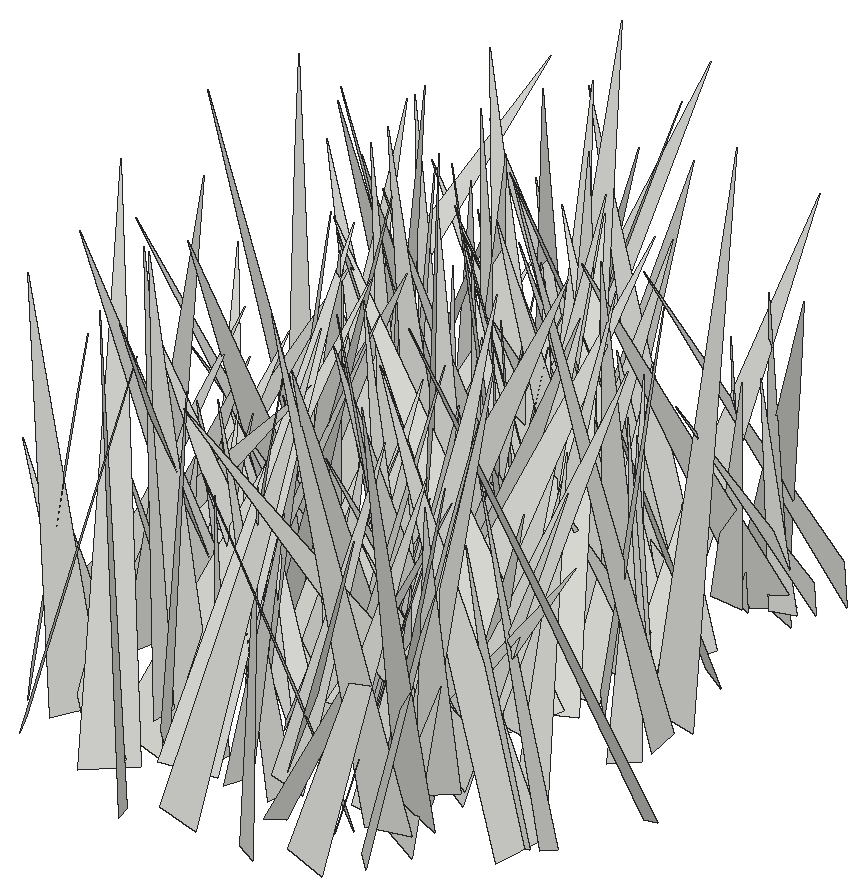
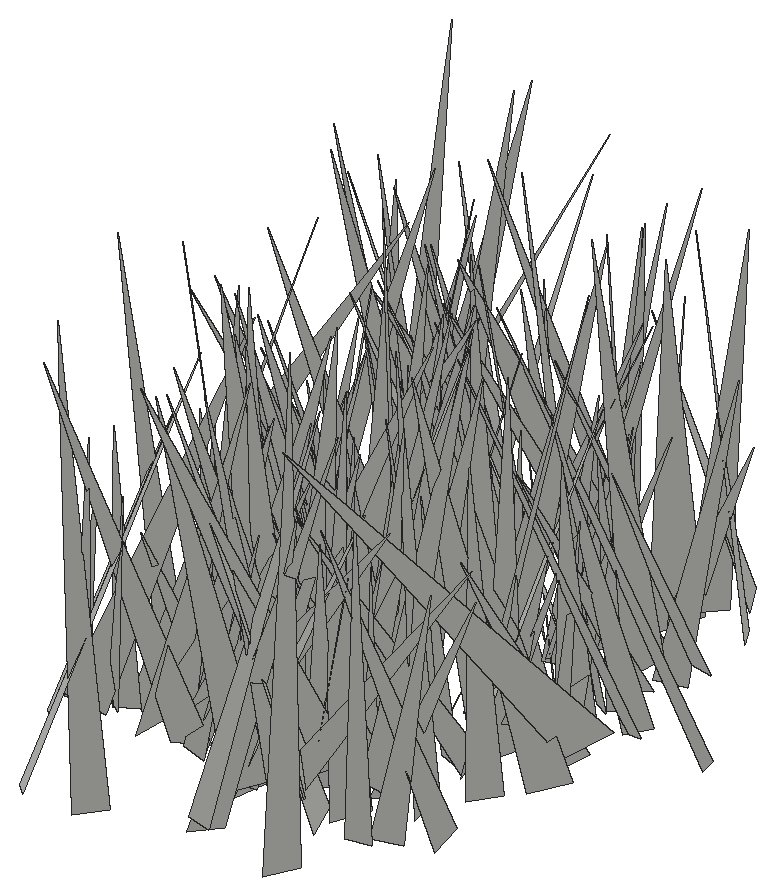
# SketchUp Ruby script. Lengths in inches.
U = 1.inch
M = Sketchup.active_model
def pt(a) = Geom::Point3d.new(a.map { |v| v * U })
def face(e, loops, mat)
  f = e.add_face(loops[0].map { |a| pt(a) })
  loops[1..].each { |l| e.add_face(l.map { |a| pt(a) }).erase! }
  f.material = f.back_material = mat if mat
  f
end
# faces: each face lists its corners as indices into pts; further lists are holes
def faces(e, pts, list, mat = nil) = list.each { |f| face(e, (f[0].is_a?(Array) ? f : [f]).map { |l| l.map { |i| pts[i] } }, mat) }
# xy, xz, yz: faces in a plane at the given z, y or x. An outline is a flat list of corners, or four numbers for a rectangle; further outlines are holes
def ring(l) = l.size == 4 ? [[l[0], l[1]], [l[2], l[1]], [l[2], l[3]], [l[0], l[3]]] : l.each_slice(2).to_a
def flat(e, list, mat, &to3) = list.each { |f| face(e, (f[0].is_a?(Array) ? f : [f]).map { |l| ring(l).map { |u, v| to3.(u, v) } }, mat) }
def xy(e, z, list, mat = nil) = flat(e, list, mat) { |x, y| [x, y, z] }
def xz(e, y, list, mat = nil) = flat(e, list, mat) { |x, z| [x, y, z] }
def yz(e, x, list, mat = nil) = flat(e, list, mat) { |y, z| [x, y, z] }
def lines(e, pts, list) = list.each { |a, b| e.add_line(pt(pts[a]), pt(pts[b])) }
# prism: a flat outline (further loops are holes) pulled along v
def prism(e, loops, v, mat = nil)
  f = face(e, loops, mat); d = Geom::Vector3d.new(v.map { |x| x * U })
  f.pushpull(f.normal.samedirection?(d) ? d.length : -d.length)
end
def box(e, o, s, mat = nil) = prism(e, [[o, [o[0] + s[0], o[1], o[2]], [o[0] + s[0], o[1] + s[1], o[2]], [o[0], o[1] + s[1], o[2]]]], [0, 0, s[2]], mat)
def at(x, y, z, deg = 0) = Geom::Transformation.translation(pt([x, y, z])) * Geom::Transformation.rotation(ORIGIN, Z_AXIS, deg.degrees)
def axes(o, x, y, z) = Geom::Transformation.new([*x, 0, *y, 0, *z, 0, *pt(o).to_a, 1])
def part(name) = M.definitions.add(name)
# library, detail: a bought-in or finely detailed component or shape, given as its bounding box
def library(name, o, s) = part(name).tap { |d| box(d.entities, o, s) }
def detail(e, o, s) = box(e.add_group.entities, o, s)
def put(e, d, t, mat = nil) = e.add_instance(d, t).tap { |i| i.material = mat if mat }
def group(e, t, mat = nil) = e.add_group.tap { |g| g.transformation = t; g.material = mat if mat }.entities
root = M.entities
c1 = part("fur_instance\#9")
p = [[0.8125,0,1.79],[0.67,-0.02,1.48],[0,-0.11,0],[0,0.11,0]]
faces(c1.entities,p,[[0,1,2,3]])
put(root,c1,axes([100.4,143.04,-28.22],[-2.55012,3.64542,1.48438],[3.93085,2.44958,0.73729],[0.20222,-1.64502,4.38733]))
put(root,c1,axes([97.49,134.62,-27.1],[1.64693,-4.65446,0.85777],[-4.4282,-1.19483,2.01879],[1.67056,1.42146,4.50564]))
put(root,c1,axes([99.8,130.2,-28.22],[2.45481,-4.16097,0.8917],[-4.06011,-2.59844,-0.9479],[-1.27449,0.26329,4.73722]))
put(root,c1,axes([99.05,135.72,-28.22],[-2.89965,3.32427,1.06428],[2.78447,3.03733,-1.90073],[2.1048,0.5615,3.98069]))
put(root,c1,axes([101.67,127.57,-28.22],[-1.66543,4.2087,0.7623],[4.0491,1.28782,1.73616],[-1.37806,-1.30242,4.18002]))
put(root,c1,axes([100.93,133.34,-28.22],[-1.93628,5.55,0.46539],[5.55779,1.89356,0.54185],[-0.36056,-0.61659,5.85304]))
put(root,c1,axes([100.48,127.66,-27.1],[-5.43342,3.18473,2.47254],[3.60205,5.6984,0.57576],[1.81141,-1.77869,6.27161]))
put(root,c1,axes([99.71,135.75,-28.22],[-0.65259,-3.58567,0.77528],[-3.62638,0.74954,0.41412],[0.55447,0.682,3.62097]))
put(root,c1,axes([98.97,132.68,-27.1],[-0.26739,4.57604,0.32256],[4.40279,0.34673,-1.26925],[1.2883,-0.2352,4.40462]))
put(root,c1,axes([101.375,137.89,-28.22],[-7.3935,-3.44968,1.78048],[-3.41196,7.60131,0.55924],[1.85173,0.23234,8.13949]))
put(root,c1,axes([98.54,128.125,-27.1],[5.36268,3.16176,1.79895],[3.56295,-5.21159,-1.4615],[-0.73371,-2.1986,6.05138]))
put(root,c1,axes([98.375,130.51,-27.1],[2.55836,5.15566,0.46861],[5.11042,-2.43162,-1.14739],[0.82709,-0.92305,5.63999]))
put(root,c1,axes([98.12,136.25,-27.1],[-4.06981,7.2471,0.38585],[5.9474,3.58401,-4.58433],[4.15906,1.9665,6.9331]))
put(root,c1,axes([102.17,135.2,-28.22],[1.13757,8.04859,1.54719],[7.76789,-1.55698,2.3882],[-2.61411,-1.12413,7.76984]))
put(root,c1,axes([101.86,127.34,-28.22],[-7.18499,4.19207,1.05141],[4.04317,7.24035,-1.23823],[1.52698,0.55406,8.22584]))
put(root,c1,axes([97.41,134.95,-27.1],[3.70489,5.29932,0.63458],[5.07029,-3.25343,-2.43293],[1.66665,-1.88258,5.99082]))
put(root,c1,axes([99.73,131.58,-27.1],[6.98669,-0.82296,2.45735],[-1.02769,-7.36659,0.45485],[-2.37901,0.76535,7.02027]))
put(root,c1,axes([99.07,141.87,-28.22],[5.64038,0.84844,0.8162],[0.68974,-5.61874,1.07421],[-0.95409,0.95384,5.60177]))
put(root,c1,axes([100.51,138.875,-27.1],[-3.99829,-3.957,0.07334],[-3.50173,3.58563,2.55553],[1.84422,-1.77059,5.01133]))
put(root,c1,axes([99.76,139.14,-28.22],[4.42383,-2.92058,1.2942],[-2.99041,-4.56361,-0.07677],[-1.12348,0.64702,5.30039]))
put(root,c1,axes([102.125,141.01,-28.22],[-3.73947,1.85603,0.44676],[1.90802,3.6015,1.00834],[-0.06253,-1.10111,4.05114]))
put(root,c1,axes([99.83,126.22,-27.1],[4.69636,2.95892,0.9191],[2.85112,-4.78039,0.82137],[-1.21287,0.21986,5.48965]))
put(root,c1,axes([99.82,145.12,-27.1],[-0.19463,-4.95849,1.24268],[-5.00803,0.4343,0.94858],[1.02496,1.18047,4.8708]))
put(root,c1,axes([99.91,132.41,-28.22],[2.26375,-3.28304,0.92587],[-3.40814,-2.22313,0.4499],[-0.14199,1.01955,3.96238]))
put(root,c1,axes([95.77,133.46,-28.22],[5.26826,5.58359,0.80335],[4.69893,-3.73546,-4.8521],[3.1212,-3.80083,5.9488]))
put(root,c1,axes([102.12,135.4,-28.22],[-3.8674,0.14725,0.40736],[0.1724,3.88071,0.23399],[0.39736,-0.25058,3.86312]))
put(root,c1,axes([101.26,142.32,-27.1],[-1.0754,-7.3325,1.08617],[-7.40599,1.10888,0.15329],[0.31086,1.05196,7.40935]))
put(root,c1,axes([103.47,136.47,-28.22],[-6.74137,-3.47517,0.05647],[-3.44773,6.70195,0.85032],[0.43951,-0.73012,7.53656]))
put(root,c1,axes([101.01,136.86,-28.22],[-5.55671,4.70477,2.20019],[4.40361,5.97611,-1.65743],[2.7539,-0.06297,7.08977]))
put(root,c1,axes([103.57,143.76,-27.1],[-0.91918,-4.72146,0.08029],[-4.18667,0.777,-2.23865],[-2.18412,0.49761,4.25741]))
put(root,c1,axes([101.43,132.44,-28.22],[-3.13954,-2.86345,1.03549],[-2.74612,3.30524,0.81394],[1.31545,0.06589,4.17056]))
put(root,c1,axes([102.83,130.66,-28.22],[-2.05485,-3.90462,0.97999],[-3.96047,1.76344,-1.27819],[-0.72186,1.43981,4.22312]))
put(root,c1,axes([102.23,132.42,-27.1],[-7.41474,-1.37074,2.09218],[-0.74138,7.45582,2.25736],[2.38883,-1.94072,7.19456]))
put(root,c1,axes([100.69,140.72,-28.22],[7.15031,1.42356,2.57616],[1.59453,-7.56218,-0.24693],[-2.47399,-0.75958,7.28646]))
put(root,c1,axes([100.49,132.67,-28.22],[2.69077,3.3772,1.27263],[3.60609,-2.57991,-0.77814],[-0.14558,-1.48455,4.24737]))
put(root,c1,axes([100.54,134.38,-28.22],[-2.64275,-7.72517,0.10148],[-7.35563,2.5487,2.46402],[2.36287,-0.70608,7.78402]))
put(root,c1,axes([101.4,136.84,-27.1],[2.31085,-7.14722,0.11909],[-7.10013,-2.30949,-0.83147],[-0.82765,-0.14321,7.46535]))
put(root,c1,axes([101.95,132.95,-27.1],[1.41164,-4.04262,0.99191],[-4.10193,-1.52908,-0.39425],[-0.70768,0.79907,4.26381]))
put(root,c1,axes([98.64,137.44,-28.22],[2.93254,-6.52755,1.0505],[-6.19008,-2.30697,2.94501],[2.32281,2.09313,6.52193]))
put(root,c1,axes([103.66,125.66,-28.22],[-6.04222,-2.58238,2.07365],[-3.21518,5.60869,-2.38377],[0.79453,3.05796,6.1233]))
put(root,c1,axes([102.47,129.28,-27.1],[-6.58404,0.20466,2.39247],[0.20033,7.00521,-0.04793],[2.39284,-0.02336,6.58705]))
put(root,c1,axes([102.99,143.48,-27.1],[-3.64875,-2.02244,1.121],[-2.25149,3.58457,-0.86132],[0.52696,1.3118,4.08188]))
put(root,c1,axes([102.81,130.24,-27.1],[-3.06168,2.49465,0.02952],[2.42804,2.99025,-0.87237],[0.57338,0.65813,3.85176]))
put(root,c1,axes([101.95,138.02,-28.22],[-1.46329,-3.87448,2.4887],[-4.52721,1.6881,-0.03379],[0.84239,2.34204,4.14146]))
put(root,c1,axes([102.71,129.72,-28.22],[-6.55699,2.55506,2.62376],[2.8465,6.94107,0.35432],[2.30431,-1.30376,7.02829]))
put(root,c1,axes([102.78,140.77,-27.1],[1.15906,3.62365,1.13013],[3.60388,-1.42153,0.86183],[-1.19166,-0.77453,3.7056]))
put(root,c1,axes([104.2,137.42,-28.22],[-6.29408,3.56033,1.19684],[3.6784,6.31519,0.55815],[0.76008,-1.07993,7.20971]))
put(root,c1,axes([100.91,138.04,-28.22],[-0.72981,5.66267,0.18679],[5.27184,0.7477,-2.06932],[2.0757,0.09199,5.32132]))
put(root,c1,axes([103.18,139.33,-27.1],[-1.62958,-3.15436,1.09529],[-3.33909,1.53504,-0.54711],[-0.01197,1.22427,3.50802]))
put(root,c1,axes([101.875,135.24,-27.1],[3.65469,-1.69105,0.3912],[-1.57801,-3.61693,-0.89287],[-0.72291,-0.65395,3.92673]))
put(root,c1,axes([104.78,132.48,-28.22],[-6.35837,1.48,1.02188],[1.69793,6.17763,1.61781],[0.593,-1.81932,6.3247]))
put(root,c1,axes([105.24,137.54,-28.22],[-7.58228,1.17889,0.51367],[1.00041,7.33787,-2.07353],[0.80796,1.97752,7.38791]))
put(root,c1,axes([103.43,141.43,-28.22],[-1.16201,-7.65185,1.0654],[-7.72512,1.16361,-0.06847],[0.09162,1.06366,7.73928]))
put(root,c1,axes([101.23,137,-27.1],[0.69431,-7.1025,1.01226],[-6.95299,-0.41552,1.85354],[1.7681,1.15502,6.89145]))
put(root,c1,axes([101.7,146.42,-28.22],[7.80174,-0.94154,1.76979],[-0.49694,-7.7978,-1.95786],[-1.94209,-1.78708,7.61055]))
put(root,c1,axes([102.625,133.17,-28.22],[0.42201,3.83383,0.13948],[3.79822,-0.3978,-0.55775],[0.53966,-0.19825,3.81644]))
put(root,c1,axes([102.2,142.51,-28.22],[6.63287,-1.89646,1.66739],[-1.83678,-6.83922,-0.47211],[-1.73291,-0.0097,6.88248]))
put(root,c1,axes([103.92,129.57,-28.22],[-3.53666,-0.44387,1.07965],[-0.6619,3.59984,-0.68824],[0.96154,0.84544,3.49732]))
put(root,c1,axes([104.36,141.24,-28.22],[-4.5808,2.50643,0.71678],[2.42315,4.62824,-0.69815],[0.96142,0.27723,5.1748]))
put(root,c1,axes([102.12,132.83,-28.22],[3.23905,1.92957,1.10614],[2.22288,-2.8741,-1.49551],[-0.07469,-1.85863,3.46094]))
put(root,c1,axes([101.57,128.9,-28.22],[0.36828,7.38641,0.21711],[7.15433,-0.30198,-1.86176],[1.84979,-0.30261,7.15741]))
put(root,c1,axes([104.59,136.19,-27.1],[3.23969,5.31398,1.47982],[4.81259,-3.56155,2.25346],[-2.69577,0.02794,5.80137]))
put(root,c1,axes([106.5,138.14,-28.22],[-7.44301,-3.63877,0.95843],[-3.76282,7.20814,-1.85509],[0.01898,2.08796,8.0745]))
put(root,c1,axes([101.47,132.19,-28.22],[4.90909,4.36789,0.50992],[4.39704,-4.86378,-0.66882],[0.06695,-0.83837,6.53684]))
put(root,c1,axes([104.47,140.68,-28.22],[-6.8831,0.44539,2.18741],[0.27023,7.20464,-0.61666],[2.21588,0.50489,6.86987]))
put(root,c1,axes([103.8,140.08,-27.1],[-0.44109,-6.89492,0.21564],[-6.89758,0.44393,0.08524],[0.09888,0.20974,6.90849]))
put(root,c1,axes([105.09,145.83,-28.22],[-6.6748,0.96554,1.83268],[1.43583,6.61336,1.7452],[1.49311,-2.0433,6.51456]))
put(root,c1,axes([107.57,141.42,-27.1],[-2.18408,5.95276,0.46734],[5.01759,1.55993,3.57972],[-3.2369,-1.59851,5.23366]))
put(root,c1,axes([105.54,144.57,-28.22],[-3.87501,-4.05549,0.17386],[-4.05477,3.85598,-0.42797],[-0.18982,0.42113,5.59281]))
put(root,c1,axes([103.8,131.41,-27.1],[4.42049,5.15695,1.86392],[5.12768,-4.73588,0.94203],[-1.94301,-0.76574,6.72662]))
put(root,c1,axes([102.46,133.34,-28.22],[7.58691,1.58366,1.76713],[1.48707,-7.78642,0.59349],[-1.84915,0.23586,7.72768]))
put(root,c1,axes([103.47,127.71,-27.1],[-3.24328,-4.06122,2.56752],[-4.33534,3.80899,0.54855],[2.07134,1.61325,5.16831]))
put(root,c1,axes([102.97,139.14,-28.22],[4.64309,0.99306,0.50279],[0.80416,-4.48393,1.43003],[-0.7696,1.30595,4.52764]))
put(root,c1,axes([105.55,143.18,-28.22],[-5.54027,1.19429,0.93196],[1.15956,5.61711,-0.30487],[0.97482,0.10593,5.65933]))
put(root,c1,axes([104.26,147.2,-27.1],[-2.87377,-5.9267,0.11201],[-5.79461,2.83495,1.33509],[1.24935,-0.48389,6.44995]))
put(root,c1,axes([105.63,131.3,-28.22],[-2.71204,2.5664,0.21286],[2.56651,2.66825,0.52947],[-0.21147,-0.53003,3.69611]))
put(root,c1,axes([105.45,140.82,-28.22],[-6.05615,5.17907,2.30301],[5.46239,6.23254,0.34836],[1.51293,-1.77094,7.96105]))
put(root,c1,axes([104.03,141.66,-28.22],[2.05705,-3.40779,1.21765],[-3.60141,-2.06493,0.30505],[-0.3543,1.20424,3.9688]))
put(root,c1,axes([105.55,136.86,-27.1],[-7.11208,1.53537,2.26223],[1.65379,7.4363,0.15223],[2.17716,-0.6331,7.27433]))
put(root,c1,axes([105.1,137.75,-28.22],[1.75124,-3.26229,0.83742],[-3.12175,-1.92651,-0.97669],[-1.26432,0.23809,3.57148]))
put(root,c1,axes([104.77,144.56,-27.1],[2.5877,-3.76016,0.15432],[-3.53923,-2.49522,-1.45139],[-1.27925,-0.70276,4.32764]))
put(root,c1,axes([104.79,127.04,-27.1],[-5.35866,5.61511,0.59327],[5.12673,5.1813,-2.73266],[2.36603,1.4904,7.2648]))
put(root,c1,axes([102.83,144.71,-27.1],[6.50661,-0.43072,0.76621],[-0.39332,-6.54513,-0.33931],[-0.78607,-0.29036,6.51202]))
put(root,c1,axes([106.34,129.06,-28.22],[-5.51822,-0.21879,0.79161],[-0.32668,5.51842,-0.75206],[0.75352,0.79022,5.4711]))
put(root,c1,axes([102.73,143.23,-28.22],[6.96857,2.87265,0.80723],[2.85827,-7.01507,0.2896],[-0.85676,-0.03815,7.53188]))
put(root,c1,axes([105.39,137.6,-28.22],[3.73526,4.02595,0.93613],[3.5763,-3.78049,1.98866],[-2.07237,0.73241,5.11915]))
put(root,c1,axes([103.26,142.21,-27.1],[-3.36255,6.42423,2.20976],[5.77924,4.00105,-2.8377],[3.57129,-0.42595,6.67271]))
put(root,c1,axes([107.63,132.94,-28.22],[-8.22184,1.12863,0.67504],[0.91948,7.98903,-2.15825],[0.94024,2.05661,8.01339]))
put(root,c1,axes([107.08,138.87,-27.1],[-4.22119,3.06488,0.48562],[3.10212,4.18863,0.52921],[0.07866,-0.71394,5.1896]))
put(root,c1,axes([105.18,137.35,-27.1],[2.53545,-3.02814,1.98338],[-3.53036,-2.60371,0.53779],[-0.80002,1.89288,3.91266]))
put(root,c1,axes([105.69,137.1,-27.1],[3.10657,-5.20372,2.6425],[-5.63717,-3.45056,-0.16782],[-1.51121,2.17421,6.05816]))
put(root,c1,axes([103.76,129.61,-28.22],[6.71325,2.37054,1.67819],[2.73448,-6.58312,-1.63968],[-0.97898,-2.13225,6.9281]))
put(root,c1,axes([105.13,132.18,-28.22],[3.51253,-2.51047,1.78394],[-2.89575,-3.6135,0.61652],[-1.0486,1.56939,4.2732]))
put(root,c1,axes([107.01,132.57,-28.22],[-4.90258,-2.23132,0.87524],[-2.28191,4.95484,-0.15015],[0.73329,0.50088,5.38438]))
put(root,c1,axes([108.45,138.17,-27.1],[-2.5015,-6.23633,1.72664],[-6.18785,1.76379,-2.59425],[-1.89304,2.47545,6.19832]))
put(root,c1,axes([105.11,132.2,-27.1],[-1.9043,4.31856,1.08738],[4.14528,2.15112,-1.28374],[1.62757,-0.42591,4.54184]))
put(root,c1,axes([105.32,130.53,-27.1],[3.38702,2.66566,0.2184],[2.51461,-3.29384,1.20529],[-0.91115,0.81867,4.13823]))
put(root,c1,axes([106.42,134.65,-28.22],[4.53456,1.85789,3.16607],[2.55783,-5.20835,-0.60709],[-2.63311,-1.85992,4.86266]))
put(root,c1,axes([106.92,140.77,-28.22],[-4.80805,-4.95386,1.3489],[-5.02147,4.92244,0.17909],[1.0701,0.84054,6.90116]))
put(root,c1,axes([105.82,143.31,-27.1],[1.37303,-5.10418,0.31363],[-5.09334,-1.39399,-0.38851],[-0.45708,0.20095,5.27134]))
put(root,c1,axes([107.87,135.82,-28.22],[-6.18556,-0.57175,1.0735],[-0.94708,5.75521,-2.39186],[0.76312,2.5082,5.73298]))
put(root,c1,axes([106.52,140.42,-28.22],[-1.18605,7.62635,1.82441],[7.84154,1.15487,0.27022],[0.00582,-1.84431,7.7133]))
put(root,c1,axes([105.04,138.09,-28.22],[0.04539,-4.24616,1.86431],[-4.44886,0.48634,1.21602],[1.30888,1.80033,4.06857]))
put(root,c1,axes([104.48,144.51,-27.1],[4.99795,-3.82327,1.26682],[-4.01963,-4.86241,1.18375],[-0.25457,1.71502,6.18026]))
put(root,c1,axes([106.47,140.75,-27.1],[5.95771,-4.00613,4.25574],[-5.13988,-6.48421,1.09155],[-2.78246,3.40011,7.09591]))
put(root,c1,axes([106.66,134.77,-27.1],[6.19858,3.66698,3.16063],[3.75526,-6.8827,0.6206],[-3.05522,-1.01998,7.17523]))
put(root,c1,axes([107.68,138.85,-28.22],[-6.32088,1.55628,0.92222],[1.03646,5.86264,-2.78949],[1.48264,2.53644,5.88169]))
put(root,c1,axes([108.74,141.95,-28.22],[-1.92463,-5.23066,1.71698],[-5.26178,1.21283,-2.20335],[-1.6191,2.27625,5.1195]))
put(root,c1,axes([108.58,136.76,-27.1],[-4.58076,1.47717,0.18742],[1.47131,4.39705,1.30451],[-0.22897,-1.29786,4.63288]))
put(root,c1,axes([105.63,138.39,-28.22],[4.05853,2.67005,1.15678],[2.78357,-4.14094,-0.20805],[-0.84796,-0.81387,4.85361]))
put(root,c1,axes([106.7,138.82,-27.1],[-3.07228,-3.20464,1.70758],[-3.41257,3.31254,0.07678],[1.24093,1.17551,4.43878]))
put(root,c1,axes([108.1,137.06,-27.1],[-5.99226,-3.56649,1.99916],[-3.93709,5.99,-1.11487],[1.10264,2.00593,6.88361]))
put(root,c1,axes([110.4,134.82,-27.1],[-5.51381,4.9525,0.02994],[4.6746,5.18943,2.47955],[-1.63592,-1.86355,6.98435]))
put(root,c1,axes([106.22,138.69,-28.22],[-4.3896,-2.50757,2.34029],[-2.3133,4.97071,0.98703],[2.5325,0.19407,4.95805]))
put(root,c1,axes([108.1,141.67,-27.1],[-4.0966,0.35691,0.30901],[0.31396,4.07547,-0.54495],[0.35257,0.51784,4.07585]))
put(root,c1,axes([106.03,137.21,-28.22],[3.89284,1.77366,0.49192],[1.64576,-3.86945,0.92782],[-0.82421,0.65077,4.17603]))
put(root,c1,axes([105.19,135.64,-28.22],[-0.9776,-5.25666,1.94415],[-5.10339,1.65068,1.89699],[2.31681,1.41798,4.99896]))
put(root,c1,axes([106.25,127.36,-27.1],[4.13039,-0.87619,1.21239],[-0.99071,-4.26996,0.28929],[-1.12075,0.54542,4.21238]))
put(root,c1,axes([106.25,124.76,-27.1],[1.83288,7.01444,0.75411],[7.05484,-1.82448,-0.17632],[-0.01908,-0.77421,7.24781]))
put(root,c1,axes([107.59,126.02,-28.22],[2.53366,4.26731,1.78001],[4.34271,-2.89305,0.75426],[-1.5872,-1.10369,4.90515]))
put(root,c1,axes([108.55,137.63,-28.22],[-4.29612,3.71614,0.38084],[3.69784,4.31285,-0.36964],[0.52979,0.03157,5.66831]))
put(root,c1,axes([108.49,140.22,-27.1],[-3.08305,4.83073,2.80211],[5.58378,2.72141,1.452],[0.09585,-3.15451,5.54372]))
put(root,c1,axes([109.32,130.875,-28.22],[-6.80477,1.06742,0.77743],[0.9228,6.76292,-1.20833],[0.94457,1.0827,6.78117]))
put(root,c1,axes([107.71,135.61,-28.22],[-4.51609,-3.87484,0.43498],[-3.47065,4.29803,2.25393],[1.77713,-1.453,5.5072]))
put(root,c1,axes([107.16,140.53,-28.22],[1.282,-6.99581,3.06835],[-7.6361,-1.26107,0.31524],[-0.21483,3.07701,7.10532]))
put(root,c1,axes([110.27,141.68,-28.22],[-7.87651,1.28049,0.44694],[1.23259,7.85729,-0.78901],[0.56579,0.70864,7.94081]))
put(root,c1,axes([104.68,135.91,-27.1],[2.05152,-6.6713,2.37008],[-6.64568,-0.96384,3.03943],[2.44098,2.98279,6.28306]))
put(root,c1,axes([109.82,140.54,-28.22],[-4.76226,4.46867,0.77555],[4.53262,4.64929,1.04363],[-0.16086,-1.29026,6.44663]))
put(root,c1,axes([108.37,129.37,-28.22],[-4.09518,-5.32392,0.52178],[-5.17841,4.11019,1.29512],[1.34181,-0.38619,6.5907]))
put(root,c1,axes([105.9,136.99,-27.1],[5.04993,-3.13211,0.88061],[-3.25342,-4.87587,1.31476],[-0.02926,1.58216,5.79512]))
put(root,c1,axes([108.86,133.51,-28.22],[1.49882,-6.76146,1.59023],[-6.75855,-1.79498,-1.262],[-1.60255,1.24632,6.80963]))
put(root,c1,axes([108.17,130.03,-27.1],[2.52886,2.74781,0.4271],[2.47453,-2.48701,1.34889],[-1.2687,0.62635,3.48225]))
put(root,c1,axes([108.3,142.4,-28.22],[-1.84979,-4.95748,0.73449],[-4.97918,1.90688,0.3307],[0.56907,0.57009,5.281]))
put(root,c1,axes([107.13,132.35,-27.1],[6.98894,-3.62557,1.01436],[-3.15649,-6.80873,-2.58782],[-2.05189,-1.87497,7.43594]))
put(root,c1,axes([106.79,139.45,-28.22],[0.03903,6.40601,1.64221],[6.43648,0.34027,-1.48032],[1.51842,-1.60705,6.23275]))
put(root,c1,axes([107.39,128.02,-27.1],[0.7475,5.23214,1.319],[5.34274,-0.53135,-0.92008],[0.75507,-1.41992,5.20456]))
put(root,c1,axes([109.97,130.86,-28.22],[-6.28358,-3.49392,1.76213],[-3.72095,6.36668,-0.64478],[1.21124,1.43309,7.16066]))
put(root,c1,axes([108.29,135.61,-27.1],[1.00933,7.00307,0.82634],[7.04916,-1.02422,0.06983],[-0.18746,-0.80782,7.07509]))
put(root,c1,axes([108.48,127.8,-27.1],[3.77258,4.9169,0.38845],[4.64704,-3.70729,1.79444],[-1.65279,0.7995,5.93196]))
put(root,c1,axes([110.65,131.89,-27.1],[-7.29463,-2.71144,0.02018],[-2.47986,6.69465,3.09773],[1.09665,-2.89718,7.13916]))
put(root,c1,axes([109.25,141.81,-27.1],[2.35364,-2.97334,1.61897],[-3.0072,-2.74184,-0.66374],[-1.55518,0.80187,3.73361]))
put(root,c1,axes([107.08,134.51,-27.1],[1.06363,7.1406,0.14161],[6.98782,-1.01087,-1.51263],[1.47601,-0.35985,7.05914]))
put(root,c1,axes([109.375,138.15,-28.22],[-0.4926,4.67354,0.05511],[4.67276,0.49124,0.10792],[-0.10156,-0.0661,4.69819]))
put(root,c1,axes([108.19,131.8,-28.22],[3.38817,-1.89067,0.4047],[-1.85762,-3.4096,-0.37677],[-0.53632,-0.13453,3.86165]))
put(root,c1,axes([106.29,129.42,-28.22],[6.71484,1.18998,0.43364],[1.2609,-6.06064,-2.89345],[0.11927,-2.92333,6.1752]))
put(root,c1,axes([108.6,128.61,-28.22],[5.00084,3.55671,0.83126],[3.26277,-4.98345,1.69387],[-1.6418,0.92989,5.89825]))
put(root,c1,axes([109.17,129.64,-28.22],[1.47589,3.3854,0.35503],[3.34161,-1.51469,0.55196],[-0.64858,-0.1002,3.65165]))
put(root,c1,axes([110.54,132.05,-27.1],[-3.53813,-0.73541,0.01575],[-0.72603,3.50386,0.50526],[0.11809,-0.49152,3.57826]))
put(root,c1,axes([109.57,140.17,-28.22],[1.52237,-3.55739,1.37163],[-3.65271,-1.78416,-0.57315],[-1.09275,1.00785,3.82677]))
put(root,c1,axes([110.48,135.39,-27.1],[-3.69849,5.78351,0.10997],[5.76561,3.69627,-0.48502],[0.46777,0.16892,6.84781]))
put(root,c1,axes([111.08,127.73,-27.1],[-1.04276,-7.37455,2.60053],[-7.71345,0.53914,-1.56404],[-1.28435,2.74945,7.28184]))
put(root,c1,axes([108.3,126.37,-27.1],[5.03908,0.51167,0.65236],[0.18588,-4.61324,2.18248],[-0.80798,2.12978,4.57066]))
put(root,c1,axes([108.6,134.73,-27.1],[3.31097,-1.72543,0.32906],[-1.73993,-3.31791,0.10944],[-0.24091,0.24944,3.73197]))
put(root,c1,axes([109.54,139.76,-28.22],[0.14601,-6.62439,2.10053],[-6.94709,-0.08453,0.21629],[0.18059,2.1039,6.62247]))
put(root,c1,axes([110.3,140.41,-28.22],[2.63611,-2.6678,0.56163],[-2.26437,-2.5776,-1.61563],[-1.51829,-0.78771,3.38467]))
put(root,c1,axes([109.13,129.71,-28.22],[0.16612,7.76506,1.97129],[7.95416,0.07536,-0.96713],[0.95574,-1.97685,7.70638]))
put(root,c1,axes([110.08,134.11,-27.1],[1.80185,5.93958,0.37976],[5.89361,-1.83593,0.75111],[-0.82954,-0.14229,6.16126]))
put(root,c1,axes([111.38,141.17,-28.22],[-3.13069,-4.74867,0.6646],[-4.79451,3.11096,-0.35688],[0.06511,0.75154,5.67659]))
put(root,c1,axes([111.46,143.64,-27.1],[1.05272,-6.58483,0.46236],[-6.33643,-1.13928,-1.79827],[-1.85027,0.15508,6.42141]))
put(root,c1,axes([108.6875,142.02,-28.22],[0.16958,6.97336,1.46095],[6.91324,0.19239,-1.72074],[1.72314,-1.45812,6.75984]))
put(root,c1,axes([110.9375,147.35,-28.22],[-5.37416,-4.85351,0.14678],[-4.51514,5.07548,2.5125],[1.7865,-1.77274,6.79157]))
put(root,c1,axes([110.43,138.99,-28.22],[-1.96871,3.37657,0.07437],[3.27614,1.93014,-0.90775],[0.82077,0.39482,3.80171]))
put(root,c1,axes([110.82,143.11,-27.1],[1.66971,3.21733,1.57549],[3.35444,-2.01427,0.55833],[-1.25742,-1.10127,3.58153]))
put(root,c1,axes([109.125,126.59,-28.22],[1.23681,5.98503,1.54047],[6.1022,-0.934,-1.27052],[0.97821,-1.7408,5.97797]))
put(root,c1,axes([109.125,133.82,-27.1],[-0.64371,5.67181,1.6895],[5.48083,1.21245,-1.9821],[2.23257,-1.34117,5.35305]))
put(root,c1,axes([110.67,144.86,-28.22],[-1.48378,-4.80354,1.85374],[-5.06695,1.70492,0.36217],[0.91449,1.65264,5.01442]))
put(root,c1,axes([113.78,136.02,-27.1],[-7.70081,-2.50661,0.76749],[-2.60656,7.57519,-1.4131],[0.27927,1.58364,7.97425]))
put(root,c1,axes([111.69,133.04,-28.22],[-4.30895,1.90574,0.59057],[1.67064,4.21479,-1.41144],[1.09067,1.07302,4.49519]))
put(root,c1,axes([108.84,132.73,-27.1],[1.93678,-3.59499,0.72466],[-3.24209,-1.29543,2.2385],[1.71404,1.61186,3.41529]))
put(root,c1,axes([109.93,131.9375,-28.22],[2.30047,4.4169,0.81433],[4.47004,-2.16262,-0.89782],[0.43686,-1.13065,4.89848]))
put(root,c1,axes([110.33,143.0625,-27.1],[0.87128,-4.23502,0.75689],[-4.24446,-0.72019,0.85631],[0.702,0.90186,4.23807]))
put(root,c1,axes([108.45,147.15,-28.22],[-0.05965,-7.49908,0.31223],[-6.76708,0.1888,3.24163],[3.24657,0.25574,6.76251]))
put(root,c1,axes([113.24,130.65,-28.22],[-7.04891,1.70289,1.4017],[1.92518,7.04086,1.12767],[1.07622,-1.44158,7.16347]))
put(root,c1,axes([109.68,129.35,-27.1],[5.83398,1.13984,1.03884],[1.35175,-5.73614,-1.2974],[-0.74243,-1.48703,5.80098]))
put(root,c1,axes([112.38,136.14,-28.22],[-4.9436,1.78617,0.77223],[1.56135,4.89918,-1.33648],[1.16143,1.01666,5.08364]))
put(root,c1,axes([113.79,131.18,-28.22],[-5.07583,-0.99149,0.0646],[-0.93064,4.62637,-2.11704],[-0.34804,2.08923,4.7186]))
put(root,c1,axes([112.24,137.05,-27.1],[0.5553,3.90242,1.15183],[3.90207,-0.84018,0.96535],[-1.15302,-0.96393,3.8217]))
put(root,c1,axes([110.39,128.99,-28.22],[3.30058,6.51639,2.13105],[6.85171,-3.21879,-0.76942],[-0.24255,-2.25268,7.26396]))
put(root,c1,axes([111.97,137.48,-27.1],[0.50374,3.60666,1.32904],[3.78488,-0.69911,0.46265],[-0.67011,-1.23747,3.61216]))
put(root,c1,axes([111.84,143.57,-27.1],[0.6335,-3.36408,1.34348],[-3.58683,-0.77327,-0.24494],[-0.50657,1.2682,3.41444]))
put(root,c1,axes([110.85,130.1,-27.1],[3.52243,-4.25283,0.7835],[-4.27225,-3.57882,-0.21878],[-0.66956,0.46198,5.5178]))
put(root,c1,axes([112.05,144.67,-27.1],[-3.67716,-3.23058,0.06887],[-2.92053,3.36739,2.02339],[1.38271,-1.47883,4.45691]))
put(root,c1,axes([111.07,128.88,-27.1],[-1.7083,-7.51191,1.45388],[-7.48357,1.95063,1.28533],[1.59333,1.10775,7.59572]))
put(root,c1,axes([112,138.7,-28.22],[2.12447,7.8086,2.15105],[8.03257,-2.31646,0.47574],[-1.03873,-1.94278,8.07844]))
put(root,c1,axes([111.57,126.04,-27.1],[4.49985,4.45709,1.03745],[4.28289,-4.6143,1.2473],[-1.61209,0.1822,6.20956]))
put(root,c1,axes([111.28,136.59,-27.1],[4.60486,4.04407,1.88978],[4.30358,-4.74303,-0.33665],[-1.18533,-1.50984,6.1193]))
put(root,c1,axes([112.99,130.82,-28.22],[-0.94166,-4.10224,1.61468],[-4.38512,0.70145,-0.77524],[-0.45421,1.73259,4.13692]))
put(root,c1,axes([116.16,132.54,-27.1],[-4.67528,-5.85921,0.505],[-5.43274,4.05599,-3.23694],[-2.25181,2.37953,6.76097]))
